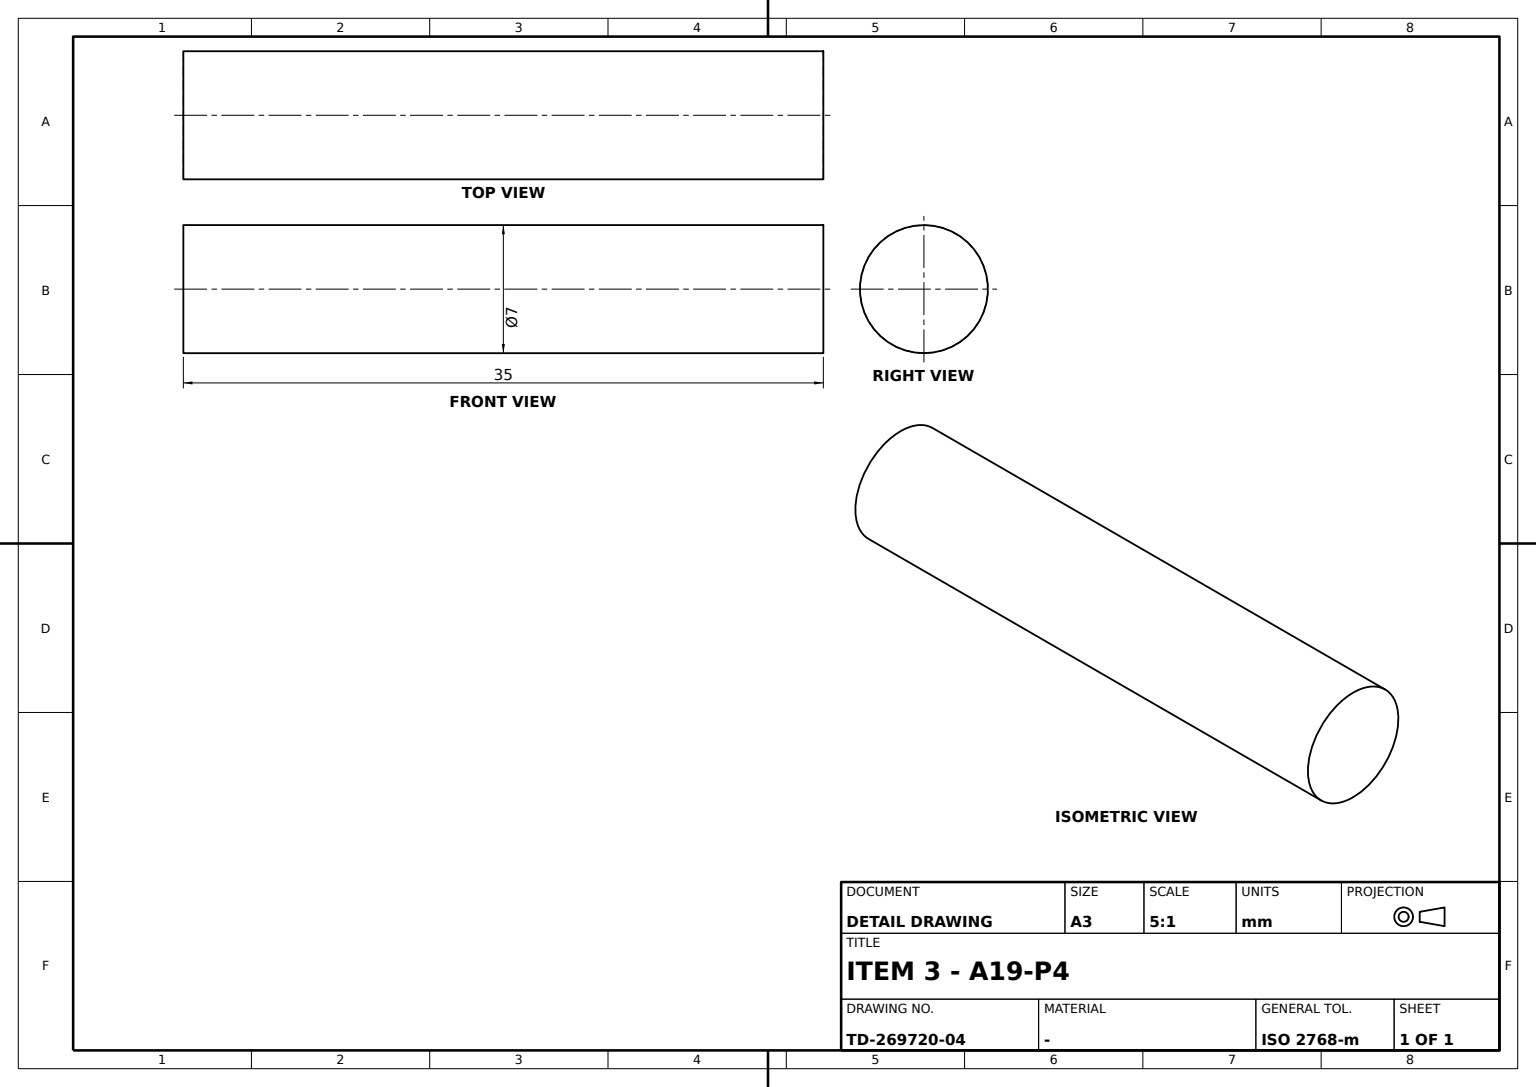
ISO-10303-21;
HEADER;
FILE_DESCRIPTION((''),'2;1');
FILE_NAME('','',(''),(''),'','','');
FILE_SCHEMA(('AUTOMOTIVE_DESIGN'));
ENDSEC;
DATA;
#1=APPLICATION_CONTEXT('');
#2=PRODUCT_CONTEXT('',#1,'mechanical');
#3=PRODUCT('','','',(#2));
#4=PRODUCT_DEFINITION_FORMATION('','',#3);
#5=PRODUCT_DEFINITION_CONTEXT('',#1,'design');
#6=PRODUCT_DEFINITION('','',#4,#5);
#7=PRODUCT_DEFINITION_SHAPE('','',#6);
#8=(LENGTH_UNIT()NAMED_UNIT(*)SI_UNIT(.MILLI.,.METRE.));
#9=(NAMED_UNIT(*)PLANE_ANGLE_UNIT()SI_UNIT($,.RADIAN.));
#10=(NAMED_UNIT(*)SI_UNIT($,.STERADIAN.)SOLID_ANGLE_UNIT());
#11=UNCERTAINTY_MEASURE_WITH_UNIT(LENGTH_MEASURE(0.005),#8,'distance_accuracy_value','');
#12=(GEOMETRIC_REPRESENTATION_CONTEXT(3)GLOBAL_UNCERTAINTY_ASSIGNED_CONTEXT((#11))GLOBAL_UNIT_ASSIGNED_CONTEXT((#8,#9,#10))REPRESENTATION_CONTEXT('',''));
#13=CARTESIAN_POINT('',(35.,0.,-3.5));
#14=VERTEX_POINT('',#13);
#15=CARTESIAN_POINT('',(35.,0.,0.));
#16=DIRECTION('',(1.,0.,0.));
#17=DIRECTION('',(0.,0.,-1.));
#18=AXIS2_PLACEMENT_3D('',#15,#16,#17);
#19=CIRCLE('',#18,3.5);
#20=EDGE_CURVE('',#14,#14,#19,.T.);
#21=ORIENTED_EDGE('',*,*,#20,.T.);
#22=EDGE_LOOP('',(#21));
#23=FACE_BOUND('',#22,.T.);
#24=DIRECTION('',(0.,1.,0.));
#25=AXIS2_PLACEMENT_3D('',#15,#16,#24);
#26=PLANE('',#25);
#27=ADVANCED_FACE('',(#23),#26,.T.);
#28=CARTESIAN_POINT('',(0.,0.,-3.5));
#29=VERTEX_POINT('',#28);
#30=CARTESIAN_POINT('',(0.,0.,0.));
#31=AXIS2_PLACEMENT_3D('',#30,#16,#17);
#32=CIRCLE('',#31,3.5);
#33=EDGE_CURVE('',#29,#29,#32,.T.);
#34=ORIENTED_EDGE('',*,*,#33,.T.);
#35=EDGE_LOOP('',(#34));
#36=FACE_BOUND('',#35,.T.);
#37=ORIENTED_EDGE('',*,*,#20,.F.);
#38=EDGE_LOOP('',(#37));
#39=FACE_BOUND('',#38,.T.);
#40=CARTESIAN_POINT('',(17.5,0.,0.));
#41=AXIS2_PLACEMENT_3D('',#40,#16,#24);
#42=CYLINDRICAL_SURFACE('',#41,3.5);
#43=ADVANCED_FACE('',(#36,#39),#42,.T.);
#44=ORIENTED_EDGE('',*,*,#33,.F.);
#45=EDGE_LOOP('',(#44));
#46=FACE_BOUND('',#45,.T.);
#47=AXIS2_PLACEMENT_3D('',#30,#16,#24);
#48=PLANE('',#47);
#49=ADVANCED_FACE('',(#46),#48,.F.);
#50=CLOSED_SHELL('',(#27,#43,#49));
#51=MANIFOLD_SOLID_BREP('',#50);
#52=ADVANCED_BREP_SHAPE_REPRESENTATION('',(#51),#12);
#53=SHAPE_DEFINITION_REPRESENTATION(#7,#52);
ENDSEC;
END-ISO-10303-21;
